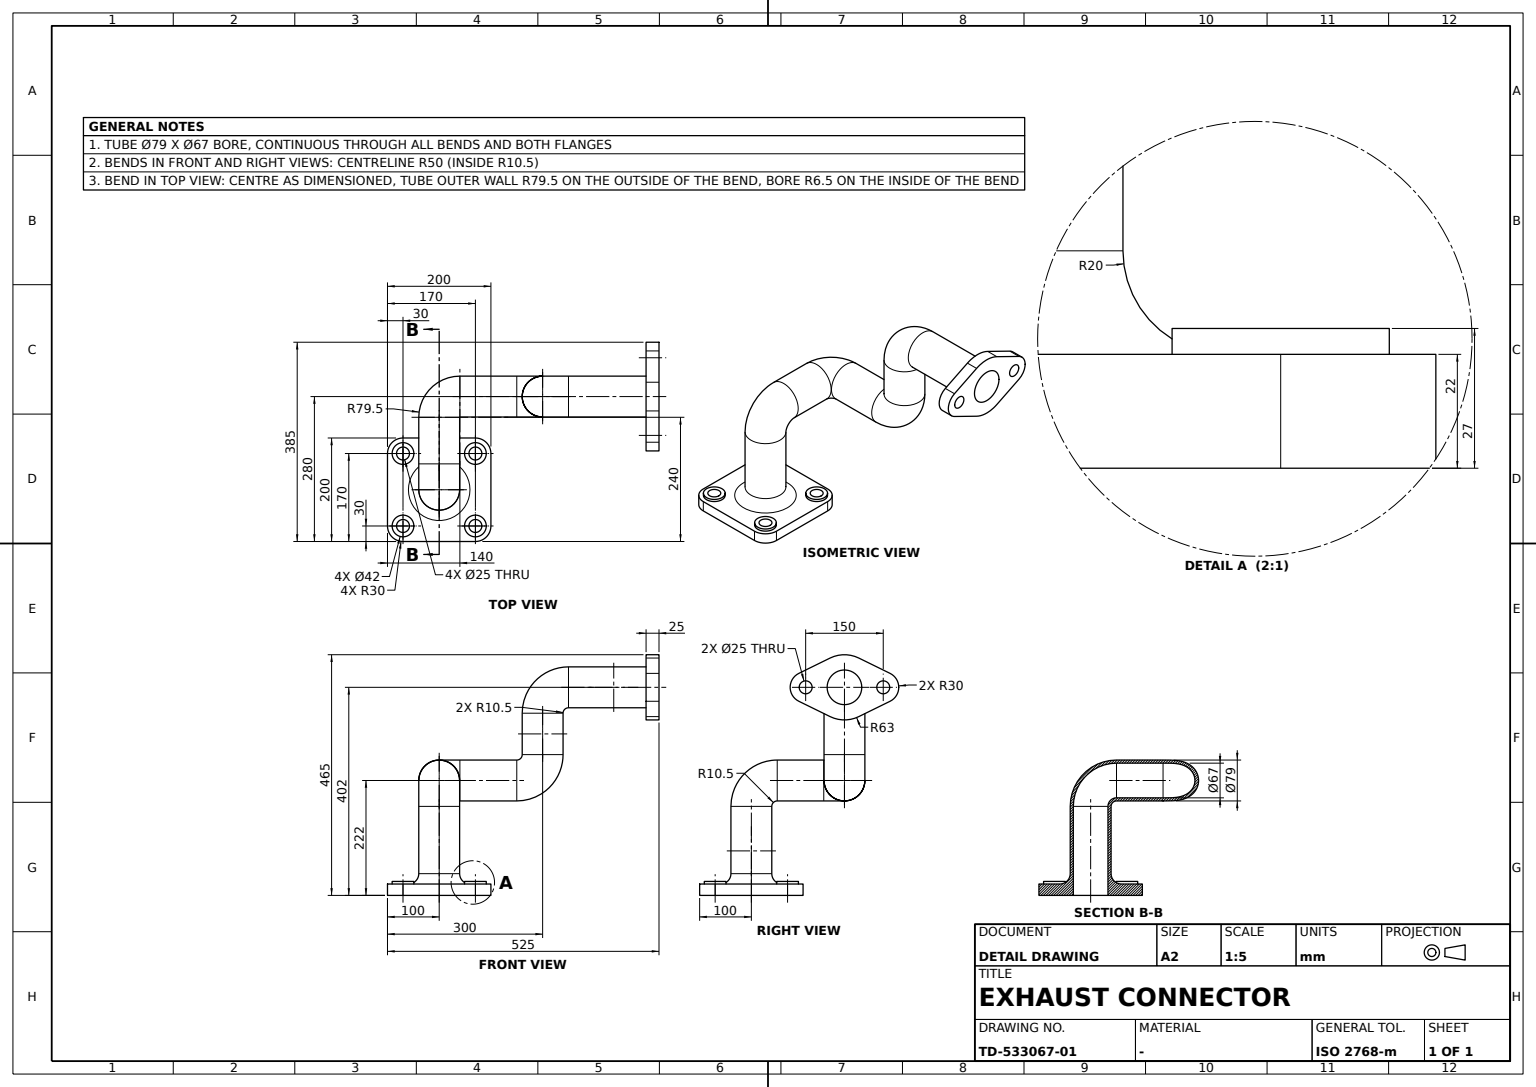
solid
v1 (-100,-70,0)
v2 (-100,70,0)
e1 v1 v2 LINE
v3 (-100,70,-22)
e2 v2 v3 LINE
v4 (-100,-70,-22)
e3 v4 v3 LINE
e4 v1 v4 LINE
face PLANE(AX(P(-100,100,0),D(1,0,0),D(0,-1,0))) rev [e1 e2 -e3 -e4]
v5 (91,70,0)
v6 (49,70,0)
e5 v5 v6 CIRCLE(AX(P(70,70,0),D(0,0,1),D(1,0,0)),21)
v7 (49,70,5)
e6 v6 v7 LINE
v8 (91,70,5)
e7 v8 v7 CIRCLE(AX(P(70,70,5),D(0,0,1),D(1,0,0)),21)
e8 v5 v8 LINE
face CYL(AX(P(70,70,2.5),D(0,0,-1),D(1,0,0)),21) [e5 e6 -e7 -e8]
v9 (400,268.2,353.060067)
v10 (400,285,380)
e9 v9 v10 CIRCLE(AX(P(400,255,380),D(1,0,0),D(0,1,0)),30)
v11 (425,285,380)
e10 v11 v10 LINE
v12 (425,268.2,353.060067)
e11 v12 v11 CIRCLE(AX(P(425,255,380),D(1,0,0),D(0,1,0)),30)
e12 v9 v12 LINE
face CYL(AX(P(412.5,255,380),D(-1,0,0),D(0,1,0)),30) [e9 -e10 -e11 -e12]
v13 (-70,100,-22)
e13 v13 v3 CIRCLE(AX(P(-70,70,-22),D(0,0,1),D(1,0,0)),30)
v14 (-70,100,0)
e14 v2 v14 CIRCLE(AX(P(-70,70,0),D(0,0,-1),D(1,0,0)),30)
e15 v14 v13 LINE
face CYL(AX(P(-70,70,-11),D(0,0,1),D(0,1,0)),30) [e13 -e2 e14 e15]
v15 (200,219.5,330)
v16 (250,219.5,380)
e16 v15 v16 CIRCLE(AX(P(250,219.5,330),D(0,1,0),D(-1,0,0)),50)
v17 (200,140.5,330)
e17 v15 v17 CIRCLE(AX(P(200,180,330),D(0,0,1),D(0,-1,0)),39.5)
v18 (250,140.5,380)
e18 v17 v18 CIRCLE(AX(P(250,140.5,330),D(0,1,0),D(-1,0,0)),50)
e19 v16 v18 CIRCLE(AX(P(250,180,380),D(1,0,0),D(0,0,1)),39.5)
face TORUS(AX(P(250,180,330),D(0,1,0),D(-1,0,0)),50,39.5) [-e16 e17 e18 -e19]
v19 (200,213.5,330)
v20 (250,213.5,380)
e20 v19 v20 CIRCLE(AX(P(250,213.5,330),D(0,1,0),D(-1,0,0)),50)
v21 (250,146.5,380)
e21 v20 v21 CIRCLE(AX(P(250,180,380),D(1,0,0),D(0,0,1)),33.5)
v22 (200,146.5,330)
e22 v22 v21 CIRCLE(AX(P(250,146.5,330),D(0,1,0),D(-1,0,0)),50)
e23 v19 v22 CIRCLE(AX(P(200,180,330),D(0,0,1),D(0,-1,0)),33.5)
face TORUS(AX(P(250,180,330),D(0,1,0),D(-1,0,0)),50,33.5) rev [e20 e21 -e22 -e23]
v23 (150,140.5,200)
v24 (150,219.5,200)
e24 v23 v24 CIRCLE(AX(P(150,180,200),D(1,0,0),D(0,0,-1)),39.5)
v25 (40,140.5,200)
e25 v25 v23 LINE
v26 (40,219.5,200)
e26 v25 v26 CIRCLE(AX(P(40,180,200),D(1,0,0),D(0,-1,0)),39.5)
e27 v26 v24 LINE
face CYL(AX(P(140.860731,180,200),D(-1,0,0),D(0,-1,0)),39.5) [-e24 -e25 e26 e27]
v27 (200,146.5,250)
e28 v27 v22 LINE
v28 (166.5,180,250)
e29 v28 v27 CIRCLE(AX(P(200,180,250),D(0,0,1),D(0,-1,0)),33.5)
v29 (200,213.5,250)
e30 v29 v28 CIRCLE(AX(P(200,180,250),D(0,0,1),D(0,-1,0)),33.5)
e31 v29 v19 LINE
face CYL(AX(P(200,180,290),D(0,0,-1),D(0,-1,0)),33.5) rev [-e28 -e29 -e30 e31 e23]
v30 (33.5,0,150)
v31 (0,33.5,150)
e32 v30 v31 CIRCLE(AX(P(0,0,150),D(0,0,1),D(0,-1,0)),33.5)
v32 (33.5,50,200)
e33 v32 v30 CIRCLE(AX(P(33.5,50,150),D(1,0,0),D(0,0,1)),50)
v33 (0,50,166.5)
e34 v32 v33 CIRCLE(AX(P(0,50,200),D(0,1,0),D(1,0,0)),33.5)
e35 v33 v31 CIRCLE(AX(P(0,50,150),D(1,0,0),D(0,0,-1)),16.5)
face TORUS(AX(P(0,50,150),D(1,0,0),D(0,0,1)),50,33.5) rev [-e32 -e33 e34 e35]
v34 (0,39.5,150)
v35 (-39.5,0,150)
e36 v34 v35 CIRCLE(AX(P(0,0,150),D(0,0,1),D(0,-1,0)),39.5)
v36 (-39.5,50,200)
e37 v36 v35 CIRCLE(AX(P(-39.5,50,150),D(1,0,0),D(0,0,1)),50)
v37 (0,50,160.5)
e38 v37 v36 CIRCLE(AX(P(0,50,200),D(0,1,0),D(1,0,0)),39.5)
e39 v37 v34 CIRCLE(AX(P(0,50,150),D(1,0,0),D(0,0,-1)),10.5)
face TORUS(AX(P(0,50,150),D(1,0,0),D(0,0,1)),50,39.5) [e36 -e37 -e38 e39]
v38 (233.5,180,330)
v39 (250,180,346.5)
e40 v38 v39 CIRCLE(AX(P(250,180,330),D(0,1,0),D(0,0,1)),16.5)
e41 v39 v20 CIRCLE(AX(P(250,180,380),D(1,0,0),D(0,0,1)),33.5)
e42 v38 v19 CIRCLE(AX(P(200,180,330),D(0,0,1),D(0,-1,0)),33.5)
face TORUS(AX(P(250,180,330),D(0,1,0),D(-1,0,0)),50,33.5) rev [e40 e41 -e20 -e42]
v40 (-59.5,0,0)
v41 (59.5,0,0)
e43 v40 v41 CIRCLE(AX(P(0,0,0),D(0,0,-1),D(1,0,0)),59.5)
v42 (-39.5,0,20)
e44 v42 v40 CIRCLE(AX(P(-59.5,0,20),D(0,1,0),D(-1,0,0)),20)
v43 (39.5,0,20)
e45 v42 v43 CIRCLE(AX(P(0,0,20),D(0,0,-1),D(1,0,0)),39.5)
e46 v43 v41 CIRCLE(AX(P(59.5,0,20),D(0,-1,0),D(1,0,0)),20)
face TORUS(AX(P(0,0,20),D(0,0,1),D(0.866025404,-0.5,0)),59.5,20) rev [-e43 -e44 e45 e46]
e47 v42 v35 LINE
v44 (39.5,0,150)
e48 v44 v34 CIRCLE(AX(P(0,0,150),D(0,0,1),D(0,-1,0)),39.5)
e49 v43 v44 LINE
face CYL(AX(P(0,0,75),D(0,0,-1),D(1,0,0)),39.5) [e47 -e36 -e48 -e49 -e45]
v45 (57.5,70,5)
v46 (57.5,70,-22)
e50 v45 v46 LINE
v47 (82.5,70,-22)
e51 v46 v47 CIRCLE(AX(P(70,70,-22),D(0,0,-1),D(1,0,0)),12.5)
v48 (82.5,70,5)
e52 v48 v47 LINE
e53 v48 v45 CIRCLE(AX(P(70,70,5),D(0,0,1),D(1,0,0)),12.5)
face CYL(AX(P(70,70,-9.16),D(0,0,-1),D(1,0,0)),12.5) rev [e50 e51 -e52 e53]
e54 v26 v25 CIRCLE(AX(P(40,180,200),D(1,0,0),D(0,-1,0)),39.5)
v49 (-39.5,140,200)
e55 v26 v49 CIRCLE(AX(P(40,140,200),D(0,0,1),D(0,1,0)),79.5)
v50 (39.5,140,200)
e56 v49 v50 CIRCLE(AX(P(0,140,200),D(0,1,0),D(1,0,0)),39.5)
e57 v25 v50 CIRCLE(AX(P(40,140,200),D(0,0,1),D(0,1,0)),0.5)
face TORUS(AX(P(40,140,200),D(0,0,1),D(0,1,0)),40,39.5) [-e54 e55 e56 -e57]
e58 v43 v42 CIRCLE(AX(P(0,0,20),D(0,0,-1),D(1,0,0)),39.5)
e59 v35 v44 CIRCLE(AX(P(0,0,150),D(0,0,1),D(0,-1,0)),39.5)
face CYL(AX(P(0,0,75),D(0,0,-1),D(1,0,0)),39.5) [-e58 e49 -e59 -e47]
v51 (400,152.28,436.57386)
v52 (425,152.28,436.57386)
e60 v51 v52 LINE
v53 (425,207.72,436.57386)
e61 v53 v52 CIRCLE(AX(P(425,180,380),D(1,0,0),D(0,1,0)),63)
v54 (400,207.72,436.57386)
e62 v54 v53 LINE
e63 v54 v51 CIRCLE(AX(P(400,180,380),D(1,0,0),D(0,1,0)),63)
face CYL(AX(P(412.5,180,380),D(-1,0,0),D(0,1,0)),63) [e60 -e61 -e62 e63]
v55 (200,219.5,250)
v56 (160.5,180,250)
e64 v55 v56 CIRCLE(AX(P(200,180,250),D(0,0,1),D(0,-1,0)),39.5)
e65 v55 v24 CIRCLE(AX(P(150,219.5,250),D(0,1,0),D(1,0,0)),50)
v57 (150,180,239.5)
e66 v24 v57 CIRCLE(AX(P(150,180,200),D(1,0,0),D(0,0,-1)),39.5)
e67 v56 v57 CIRCLE(AX(P(150,180,250),D(0,1,0),D(0,0,1)),10.5)
face TORUS(AX(P(150,180,250),D(0,1,0),D(1,0,0)),50,39.5) [-e64 e65 e66 -e67]
v58 (40,213.5,200)
v59 (-33.5,140,200)
e68 v58 v59 CIRCLE(AX(P(40,140,200),D(0,0,1),D(0,1,0)),73.5)
v60 (33.5,140,200)
e69 v60 v59 CIRCLE(AX(P(0,140,200),D(0,1,0),D(1,0,0)),33.5)
v61 (40,146.5,200)
e70 v61 v60 CIRCLE(AX(P(40,140,200),D(0,0,1),D(0,1,0)),6.5)
e71 v61 v58 CIRCLE(AX(P(40,180,200),D(1,0,0),D(0,-1,0)),33.5)
face TORUS(AX(P(40,140,200),D(0,0,1),D(0,1,0)),40,33.5) rev [e68 -e69 -e70 e71]
v62 (425,146.5,380)
v63 (425,213.5,380)
e72 v62 v63 CIRCLE(AX(P(425,180,380),D(1,0,0),D(0,1,0)),33.5)
v64 (400,213.5,380)
e73 v64 v63 LINE
v65 (400,146.5,380)
e74 v65 v64 CIRCLE(AX(P(400,180,380),D(1,0,0),D(0,1,0)),33.5)
e75 v65 v62 LINE
face CYL(AX(P(412.5,180,380),D(-1,0,0),D(0,1,0)),33.5) rev [e72 -e73 -e74 e75]
v66 (-82.5,-70,5)
v67 (-57.5,-70,5)
e76 v66 v67 CIRCLE(AX(P(-70,-70,5),D(0,0,1),D(1,0,0)),12.5)
v68 (-57.5,-70,-22)
e77 v67 v68 LINE
v69 (-82.5,-70,-22)
e78 v68 v69 CIRCLE(AX(P(-70,-70,-22),D(0,0,-1),D(1,0,0)),12.5)
e79 v66 v69 LINE
face CYL(AX(P(-70,-70,-9.16),D(0,0,-1),D(1,0,0)),12.5) rev [e76 e77 e78 -e79]
v70 (91,-70,0)
v71 (49,-70,0)
e80 v70 v71 CIRCLE(AX(P(70,-70,0),D(0,0,1),D(1,0,0)),21)
v72 (49,-70,5)
e81 v71 v72 LINE
v73 (91,-70,5)
e82 v73 v72 CIRCLE(AX(P(70,-70,5),D(0,0,1),D(1,0,0)),21)
e83 v70 v73 LINE
face CYL(AX(P(70,-70,2.5),D(0,0,-1),D(1,0,0)),21) [e80 e81 -e82 -e83]
v74 (70,-100,0)
v75 (70,-100,-22)
e84 v74 v75 LINE
v76 (100,-70,-22)
e85 v75 v76 CIRCLE(AX(P(70,-70,-22),D(0,0,1),D(1,0,0)),30)
v77 (100,-70,0)
e86 v77 v76 LINE
e87 v77 v74 CIRCLE(AX(P(70,-70,0),D(0,0,-1),D(1,0,0)),30)
face CYL(AX(P(70,-70,-11),D(0,0,1),D(0,-1,0)),30) [e84 e85 -e86 e87]
v78 (425,91.8,406.939933)
e88 v52 v78 LINE
v79 (400,91.8,406.939933)
e89 v51 v79 LINE
e90 v79 v78 LINE
face PLANE(AX(P(400,91.8,406.939933),D(0,0.44,-0.897997773),D(0,0.897997773,0.44))) rev [-e88 -e60 e89 e90]
v80 (400,219.5,380)
v81 (400,140.5,380)
e91 v80 v81 CIRCLE(AX(P(400,180,380),D(1,0,0),D(0,-1,0)),39.5)
e92 v16 v80 LINE
e93 v18 v81 LINE
face CYL(AX(P(325,180,380),D(-1,0,0),D(0,-1,0)),39.5) [-e91 -e92 e19 e93]
v82 (33.5,0,-22)
e94 v82 v30 LINE
v83 (-33.5,0,150)
e95 v31 v83 CIRCLE(AX(P(0,0,150),D(0,0,1),D(0,-1,0)),33.5)
v84 (-33.5,0,-22)
e96 v83 v84 LINE
e97 v84 v82 CIRCLE(AX(P(0,0,-22),D(0,0,-1),D(1,0,0)),33.5)
face CYL(AX(P(0,0,-11),D(0,0,1),D(1,0,0)),33.5) rev [e94 e32 e95 e96 e97]
v85 (-91,-70,5)
v86 (-49,-70,5)
e98 v85 v86 CIRCLE(AX(P(-70,-70,5),D(0,0,1),D(1,0,0)),21)
v87 (-91,-70,0)
e99 v87 v85 LINE
v88 (-49,-70,0)
e100 v87 v88 CIRCLE(AX(P(-70,-70,0),D(0,0,1),D(1,0,0)),21)
e101 v88 v86 LINE
face CYL(AX(P(-70,-70,2.5),D(0,0,-1),D(1,0,0)),21) [-e98 -e99 e100 e101]
v89 (239.5,180,330)
e102 v17 v89 CIRCLE(AX(P(200,180,330),D(0,0,1),D(0,-1,0)),39.5)
v90 (250,180,340.5)
e103 v89 v90 CIRCLE(AX(P(250,180,330),D(0,1,0),D(0,0,1)),10.5)
e104 v18 v90 CIRCLE(AX(P(250,180,380),D(1,0,0),D(0,0,1)),39.5)
face TORUS(AX(P(250,180,330),D(0,1,0),D(-1,0,0)),50,39.5) [-e18 e102 e103 -e104]
e105 v90 v16 CIRCLE(AX(P(250,180,380),D(1,0,0),D(0,0,1)),39.5)
e106 v81 v80 CIRCLE(AX(P(400,180,380),D(1,0,0),D(0,-1,0)),39.5)
face CYL(AX(P(325,180,380),D(-1,0,0),D(0,-1,0)),39.5) [-e93 e104 e105 e92 -e106]
v91 (400,92.5,380)
v92 (400,117.5,380)
e107 v91 v92 CIRCLE(AX(P(400,105,380),D(1,0,0),D(0,-1,0)),12.5)
v93 (425,92.5,380)
e108 v93 v91 LINE
v94 (425,117.5,380)
e109 v93 v94 CIRCLE(AX(P(425,105,380),D(1,0,0),D(0,1,0)),12.5)
e110 v94 v92 LINE
face CYL(AX(P(161.84,105,380),D(-1,0,0),D(0,1,0)),12.5) rev [-e107 -e108 e109 e110]
v95 (-91,70,5)
v96 (-49,70,5)
e111 v95 v96 CIRCLE(AX(P(-70,70,5),D(0,0,1),D(1,0,0)),21)
v97 (-91,70,0)
e112 v97 v95 LINE
v98 (-49,70,0)
e113 v97 v98 CIRCLE(AX(P(-70,70,0),D(0,0,1),D(1,0,0)),21)
e114 v98 v96 LINE
face CYL(AX(P(-70,70,2.5),D(0,0,-1),D(1,0,0)),21) [-e111 -e112 e113 e114]
e115 v27 v29 CIRCLE(AX(P(200,180,250),D(0,0,1),D(0,-1,0)),33.5)
e116 v22 v38 CIRCLE(AX(P(200,180,330),D(0,0,1),D(0,-1,0)),33.5)
face CYL(AX(P(200,180,290),D(0,0,-1),D(0,-1,0)),33.5) rev [-e115 e28 e116 e42 -e31]
e117 v36 v49 LINE
v99 (39.5,50,200)
e118 v36 v99 CIRCLE(AX(P(0,50,200),D(0,1,0),D(1,0,0)),39.5)
e119 v99 v50 LINE
face CYL(AX(P(0,95,200),D(0,-1,0),D(1,0,0)),39.5) [-e56 -e117 e118 e119]
v100 (-33.5,50,200)
e120 v100 v59 LINE
e121 v33 v100 CIRCLE(AX(P(0,50,200),D(0,1,0),D(1,0,0)),33.5)
e122 v32 v60 LINE
face CYL(AX(P(0,95,200),D(0,-1,0),D(1,0,0)),33.5) rev [-e120 -e121 -e34 e122 e69]
e123 v99 v44 CIRCLE(AX(P(39.5,50,150),D(1,0,0),D(0,0,1)),50)
face TORUS(AX(P(0,50,150),D(1,0,0),D(0,0,1)),50,39.5) [-e123 -e118 e37 e59]
v101 (425,207.72,323.42614)
e124 v101 v12 LINE
v102 (400,207.72,323.42614)
e125 v102 v101 LINE
e126 v102 v9 LINE
face PLANE(AX(P(400,207.72,323.42614),D(0,0.44,-0.897997773),D(0,0.897997773,0.44))) [-e124 -e125 e126 e12]
e127 v96 v95 CIRCLE(AX(P(-70,70,5),D(0,0,1),D(1,0,0)),21)
e128 v98 v97 CIRCLE(AX(P(-70,70,0),D(0,0,1),D(1,0,0)),21)
face CYL(AX(P(-70,70,2.5),D(0,0,-1),D(1,0,0)),21) [-e127 -e114 e128 e112]
v103 (400,268.2,406.939933)
v104 (425,268.2,406.939933)
e129 v103 v104 LINE
e130 v11 v104 CIRCLE(AX(P(425,255,380),D(1,0,0),D(0,1,0)),30)
e131 v10 v103 CIRCLE(AX(P(400,255,380),D(1,0,0),D(0,1,0)),30)
face CYL(AX(P(412.5,255,380),D(-1,0,0),D(0,1,0)),30) [e129 -e130 e10 e131]
e132 v94 v93 CIRCLE(AX(P(425,105,380),D(1,0,0),D(0,1,0)),12.5)
e133 v92 v91 CIRCLE(AX(P(400,105,380),D(1,0,0),D(0,-1,0)),12.5)
face CYL(AX(P(161.84,105,380),D(-1,0,0),D(0,1,0)),12.5) rev [e132 e108 -e133 -e110]
e134 v41 v40 CIRCLE(AX(P(0,0,0),D(0,0,-1),D(1,0,0)),59.5)
face TORUS(AX(P(0,0,20),D(0,0,1),D(-0.5,0.866025404,0)),59.5,20) rev [e58 e44 -e134 -e46]
v105 (57.5,-70,5)
v106 (82.5,-70,5)
e135 v105 v106 CIRCLE(AX(P(70,-70,5),D(0,0,1),D(1,0,0)),12.5)
e136 v106 v105 CIRCLE(AX(P(70,-70,5),D(0,0,1),D(1,0,0)),12.5)
e137 v72 v73 CIRCLE(AX(P(70,-70,5),D(0,0,1),D(1,0,0)),21)
face PLANE(AX(P(0,0,5),D(0,0,1),D(1,0,0))) [-e135 -e136] [e137 e82]
v107 (400,152.28,323.42614)
e138 v107 v102 CIRCLE(AX(P(400,180,380),D(1,0,0),D(0,1,0)),63)
v108 (425,152.28,323.42614)
e139 v108 v101 CIRCLE(AX(P(425,180,380),D(1,0,0),D(0,1,0)),63)
e140 v107 v108 LINE
face CYL(AX(P(412.5,180,380),D(-1,0,0),D(0,1,0)),63) [e138 e125 -e139 -e140]
v109 (425,267.5,380)
v110 (425,242.5,380)
e141 v109 v110 CIRCLE(AX(P(425,255,380),D(1,0,0),D(0,1,0)),12.5)
e142 v110 v109 CIRCLE(AX(P(425,255,380),D(1,0,0),D(0,1,0)),12.5)
e143 v63 v62 CIRCLE(AX(P(425,180,380),D(1,0,0),D(0,1,0)),33.5)
v111 (425,91.8,353.060067)
e144 v78 v111 CIRCLE(AX(P(425,105,380),D(1,0,0),D(0,1,0)),30)
e145 v111 v108 LINE
e146 v104 v53 LINE
face PLANE(AX(P(425,0,0),D(1,0,0),D(0,1,0))) [-e109 -e132] [-e141 -e142] [-e72 -e143] [e88 e144 e145 e139 e124 e11 e130 e146 e61]
v112 (-57.5,70,5)
v113 (-57.5,70,-22)
e147 v112 v113 LINE
v114 (-82.5,70,5)
e148 v112 v114 CIRCLE(AX(P(-70,70,5),D(0,0,1),D(1,0,0)),12.5)
v115 (-82.5,70,-22)
e149 v114 v115 LINE
e150 v115 v113 CIRCLE(AX(P(-70,70,-22),D(0,0,-1),D(1,0,0)),12.5)
face CYL(AX(P(-70,70,-9.16),D(0,0,-1),D(1,0,0)),12.5) rev [-e147 e148 e149 e150]
v116 (200,140.5,250)
e151 v56 v116 CIRCLE(AX(P(200,180,250),D(0,0,1),D(0,-1,0)),39.5)
e152 v116 v17 LINE
e153 v55 v15 LINE
face CYL(AX(P(200,180,290),D(0,0,-1),D(0,-1,0)),39.5) [e151 e152 -e17 -e153 e64]
e154 v71 v70 CIRCLE(AX(P(70,-70,0),D(0,0,1),D(1,0,0)),21)
face CYL(AX(P(70,-70,2.5),D(0,0,-1),D(1,0,0)),21) [-e81 e154 e83 -e137]
v117 (400,91.8,353.060067)
e155 v79 v117 CIRCLE(AX(P(400,105,380),D(1,0,0),D(0,1,0)),30)
e156 v117 v111 LINE
face CYL(AX(P(412.5,105,380),D(-1,0,0),D(0,1,0)),30) [e155 e156 -e144 -e90]
e157 v100 v83 CIRCLE(AX(P(-33.5,50,150),D(1,0,0),D(0,0,1)),50)
face TORUS(AX(P(0,50,150),D(1,0,0),D(0,0,1)),50,33.5) rev [-e35 e121 e157 -e95]
v118 (100,70,-22)
e158 v118 v76 LINE
v119 (100,70,0)
e159 v119 v118 LINE
e160 v119 v77 LINE
face PLANE(AX(P(100,-100,0),D(-1,0,0),D(0,1,0))) rev [-e158 -e159 e160 e86]
e161 v69 v68 CIRCLE(AX(P(-70,-70,-22),D(0,0,-1),D(1,0,0)),12.5)
e162 v67 v66 CIRCLE(AX(P(-70,-70,5),D(0,0,1),D(1,0,0)),12.5)
face CYL(AX(P(-70,-70,-9.16),D(0,0,-1),D(1,0,0)),12.5) rev [e79 e161 -e77 e162]
e163 v57 v23 CIRCLE(AX(P(150,180,200),D(1,0,0),D(0,0,-1)),39.5)
face CYL(AX(P(140.860731,180,200),D(-1,0,0),D(0,-1,0)),39.5) [e25 -e163 -e66 -e27 e54]
e164 v103 v54 LINE
face PLANE(AX(P(400,207.72,436.57386),D(0,-0.44,-0.897997773),D(0,0.897997773,-0.44))) rev [-e146 -e129 e164 e62]
e165 v59 v60 CIRCLE(AX(P(0,140,200),D(0,1,0),D(1,0,0)),33.5)
e166 v58 v61 CIRCLE(AX(P(40,180,200),D(1,0,0),D(0,-1,0)),33.5)
face TORUS(AX(P(40,140,200),D(0,0,1),D(0,1,0)),40,33.5) rev [e70 -e165 -e68 e166]
v120 (150,146.5,200)
e167 v61 v120 LINE
v121 (150,213.5,200)
e168 v120 v121 CIRCLE(AX(P(150,180,200),D(1,0,0),D(0,0,-1)),33.5)
e169 v58 v121 LINE
face CYL(AX(P(140.860731,180,200),D(-1,0,0),D(0,-1,0)),33.5) rev [-e71 e167 e168 -e169]
e170 v45 v48 CIRCLE(AX(P(70,70,5),D(0,0,1),D(1,0,0)),12.5)
e171 v7 v8 CIRCLE(AX(P(70,70,5),D(0,0,1),D(1,0,0)),21)
face PLANE(AX(P(0,0,5),D(0,0,1),D(1,0,0))) [-e53 -e170] [e7 e171]
e172 v20 v64 LINE
e173 v64 v65 CIRCLE(AX(P(400,180,380),D(1,0,0),D(0,1,0)),33.5)
e174 v21 v65 LINE
face CYL(AX(P(325,180,380),D(-1,0,0),D(0,-1,0)),33.5) rev [e172 e173 -e174 -e21]
e175 v117 v107 LINE
face PLANE(AX(P(400,91.8,353.060067),D(0,-0.44,-0.897997773),D(0,0.897997773,-0.44))) [e140 -e145 -e156 e175]
e176 v114 v112 CIRCLE(AX(P(-70,70,5),D(0,0,1),D(1,0,0)),12.5)
face PLANE(AX(P(0,0,5),D(0,0,1),D(1,0,0))) [e111 e127] [-e176 -e148]
e177 v6 v5 CIRCLE(AX(P(70,70,0),D(0,0,1),D(1,0,0)),21)
v122 (70,100,0)
e178 v122 v119 CIRCLE(AX(P(70,70,0),D(0,0,-1),D(1,0,0)),30)
e179 v14 v122 LINE
v123 (-70,-100,0)
e180 v123 v1 CIRCLE(AX(P(-70,-70,0),D(0,0,-1),D(1,0,0)),30)
e181 v74 v123 LINE
e182 v88 v87 CIRCLE(AX(P(-70,-70,0),D(0,0,1),D(1,0,0)),21)
face PLANE(AX(P(0,0,0),D(0,0,1),D(1,0,0))) [-e113 -e128] [e134 e43] [-e5 -e177] [-e80 -e154] [-e178 -e179 -e14 -e1 -e180 -e181 -e87 -e160] [-e182 -e100]
v124 (70,100,-22)
e183 v122 v124 LINE
e184 v13 v124 LINE
face PLANE(AX(P(100,100,0),D(0,-1,0),D(-1,0,0))) rev [e183 -e184 -e15 e179]
e185 v47 v46 CIRCLE(AX(P(70,70,-22),D(0,0,-1),D(1,0,0)),12.5)
face CYL(AX(P(70,70,-9.16),D(0,0,-1),D(1,0,0)),12.5) rev [e185 -e50 e170 e52]
v125 (150,180,233.5)
e186 v121 v125 CIRCLE(AX(P(150,180,200),D(1,0,0),D(0,0,-1)),33.5)
e187 v125 v120 CIRCLE(AX(P(150,180,200),D(1,0,0),D(0,0,-1)),33.5)
face CYL(AX(P(140.860731,180,200),D(-1,0,0),D(0,-1,0)),33.5) rev [-e167 -e166 e169 e186 e187]
e188 v100 v32 CIRCLE(AX(P(0,50,200),D(0,1,0),D(1,0,0)),33.5)
face CYL(AX(P(0,95,200),D(0,-1,0),D(1,0,0)),33.5) rev [-e188 e120 e165 -e122]
e189 v21 v39 CIRCLE(AX(P(250,180,380),D(1,0,0),D(0,0,1)),33.5)
face TORUS(AX(P(250,180,330),D(0,1,0),D(-1,0,0)),50,33.5) rev [e22 e189 -e40 -e116]
e190 v29 v121 CIRCLE(AX(P(150,213.5,250),D(0,1,0),D(1,0,0)),50)
e191 v27 v120 CIRCLE(AX(P(150,146.5,250),D(0,1,0),D(1,0,0)),50)
face TORUS(AX(P(150,180,250),D(0,1,0),D(1,0,0)),50,33.5) rev [e115 e190 -e168 -e191]
v126 (400,267.5,380)
v127 (400,242.5,380)
e192 v126 v127 CIRCLE(AX(P(400,255,380),D(1,0,0),D(0,-1,0)),12.5)
e193 v109 v126 LINE
e194 v110 v127 LINE
face CYL(AX(P(161.84,255,380),D(-1,0,0),D(0,1,0)),12.5) rev [-e192 -e193 e141 e194]
v128 (57.5,-70,-22)
v129 (82.5,-70,-22)
e195 v128 v129 CIRCLE(AX(P(70,-70,-22),D(0,0,-1),D(1,0,0)),12.5)
e196 v129 v128 CIRCLE(AX(P(70,-70,-22),D(0,0,-1),D(1,0,0)),12.5)
e197 v113 v115 CIRCLE(AX(P(-70,70,-22),D(0,0,-1),D(1,0,0)),12.5)
e198 v82 v84 CIRCLE(AX(P(0,0,-22),D(0,0,-1),D(1,0,0)),33.5)
e199 v118 v124 CIRCLE(AX(P(70,70,-22),D(0,0,1),D(1,0,0)),30)
v130 (-70,-100,-22)
e200 v75 v130 LINE
e201 v4 v130 CIRCLE(AX(P(-70,-70,-22),D(0,0,1),D(1,0,0)),30)
face PLANE(AX(P(0,0,-22),D(0,0,-1),D(1,0,0))) [-e195 -e196] [-e197 -e150] [-e161 -e78] [-e198 -e97] [-e51 -e185] [e3 -e13 e184 -e199 e158 -e85 e200 -e201]
e202 v28 v125 CIRCLE(AX(P(150,180,250),D(0,1,0),D(0,0,1)),16.5)
face TORUS(AX(P(150,180,250),D(0,1,0),D(1,0,0)),50,33.5) rev [-e202 e29 e191 -e187]
e203 v116 v55 CIRCLE(AX(P(200,180,250),D(0,0,1),D(0,-1,0)),39.5)
e204 v89 v15 CIRCLE(AX(P(200,180,330),D(0,0,1),D(0,-1,0)),39.5)
face CYL(AX(P(200,180,290),D(0,0,-1),D(0,-1,0)),39.5) [-e152 e203 e153 -e204 -e102]
face TORUS(AX(P(150,180,250),D(0,1,0),D(1,0,0)),50,33.5) rev [e202 -e186 -e190 e30]
e205 v99 v37 CIRCLE(AX(P(0,50,200),D(0,1,0),D(1,0,0)),39.5)
e206 v50 v49 CIRCLE(AX(P(0,140,200),D(0,1,0),D(1,0,0)),39.5)
face CYL(AX(P(0,95,200),D(0,-1,0),D(1,0,0)),39.5) [-e119 e205 e38 e117 -e206]
e207 v83 v30 CIRCLE(AX(P(0,0,150),D(0,0,1),D(0,-1,0)),33.5)
face TORUS(AX(P(0,50,150),D(1,0,0),D(0,0,1)),50,33.5) rev [e33 -e207 -e157 e188]
e208 v116 v23 CIRCLE(AX(P(150,140.5,250),D(0,1,0),D(1,0,0)),50)
face TORUS(AX(P(150,180,250),D(0,1,0),D(1,0,0)),50,39.5) [-e203 e208 e24 -e65]
face CYL(AX(P(412.5,180,380),D(-1,0,0),D(0,1,0)),33.5) rev [e73 e143 -e75 -e173]
face TORUS(AX(P(150,180,250),D(0,1,0),D(1,0,0)),50,39.5) [-e208 -e151 e67 e163]
e209 v123 v130 LINE
face PLANE(AX(P(-100,-100,0),D(0,1,0),D(1,0,0))) rev [-e84 e181 e209 -e200]
face TORUS(AX(P(0,50,150),D(1,0,0),D(0,0,1)),50,39.5) [e48 -e39 -e205 e123]
e210 v86 v85 CIRCLE(AX(P(-70,-70,5),D(0,0,1),D(1,0,0)),21)
face CYL(AX(P(-70,-70,2.5),D(0,0,-1),D(1,0,0)),21) [e99 -e210 -e101 e182]
e211 v105 v128 LINE
e212 v106 v129 LINE
face CYL(AX(P(70,-70,-9.16),D(0,0,-1),D(1,0,0)),12.5) rev [-e211 e135 e212 e196]
e213 v127 v126 CIRCLE(AX(P(400,255,380),D(1,0,0),D(0,-1,0)),12.5)
face PLANE(AX(P(400,180,380),D(1,0,0),D(0,-1,0))) rev [e107 e133] [e91 e106] [e192 e213] [-e175 -e155 -e89 -e63 -e164 -e131 -e9 -e126 -e138]
face CYL(AX(P(325,180,380),D(-1,0,0),D(0,-1,0)),33.5) rev [-e172 -e41 -e189 e174 e74]
face CYL(AX(P(-70,70,-9.16),D(0,0,-1),D(1,0,0)),12.5) rev [e176 e147 e197 -e149]
face TORUS(AX(P(250,180,330),D(0,1,0),D(-1,0,0)),50,39.5) [-e103 e204 e16 -e105]
face PLANE(AX(P(0,0,5),D(0,0,1),D(1,0,0))) [-e76 -e162] [e98 e210]
face CYL(AX(P(70,70,-11),D(0,0,1),D(1,0,0)),30) [e178 e159 e199 -e183]
face CYL(AX(P(70,70,2.5),D(0,0,-1),D(1,0,0)),21) [e177 e8 -e171 -e6]
face CYL(AX(P(-70,-70,-11),D(0,0,1),D(-1,0,0)),30) [-e209 e180 e4 e201]
face TORUS(AX(P(40,140,200),D(0,0,1),D(0,1,0)),40,39.5) [e206 -e55 -e26 e57]
face CYL(AX(P(70,-70,-9.16),D(0,0,-1),D(1,0,0)),12.5) rev [e136 e211 e195 -e212]
face CYL(AX(P(0,0,-11),D(0,0,1),D(1,0,0)),33.5) rev [-e96 e207 -e94 e198]
face CYL(AX(P(161.84,255,380),D(-1,0,0),D(0,1,0)),12.5) rev [-e213 -e194 e142 e193]
